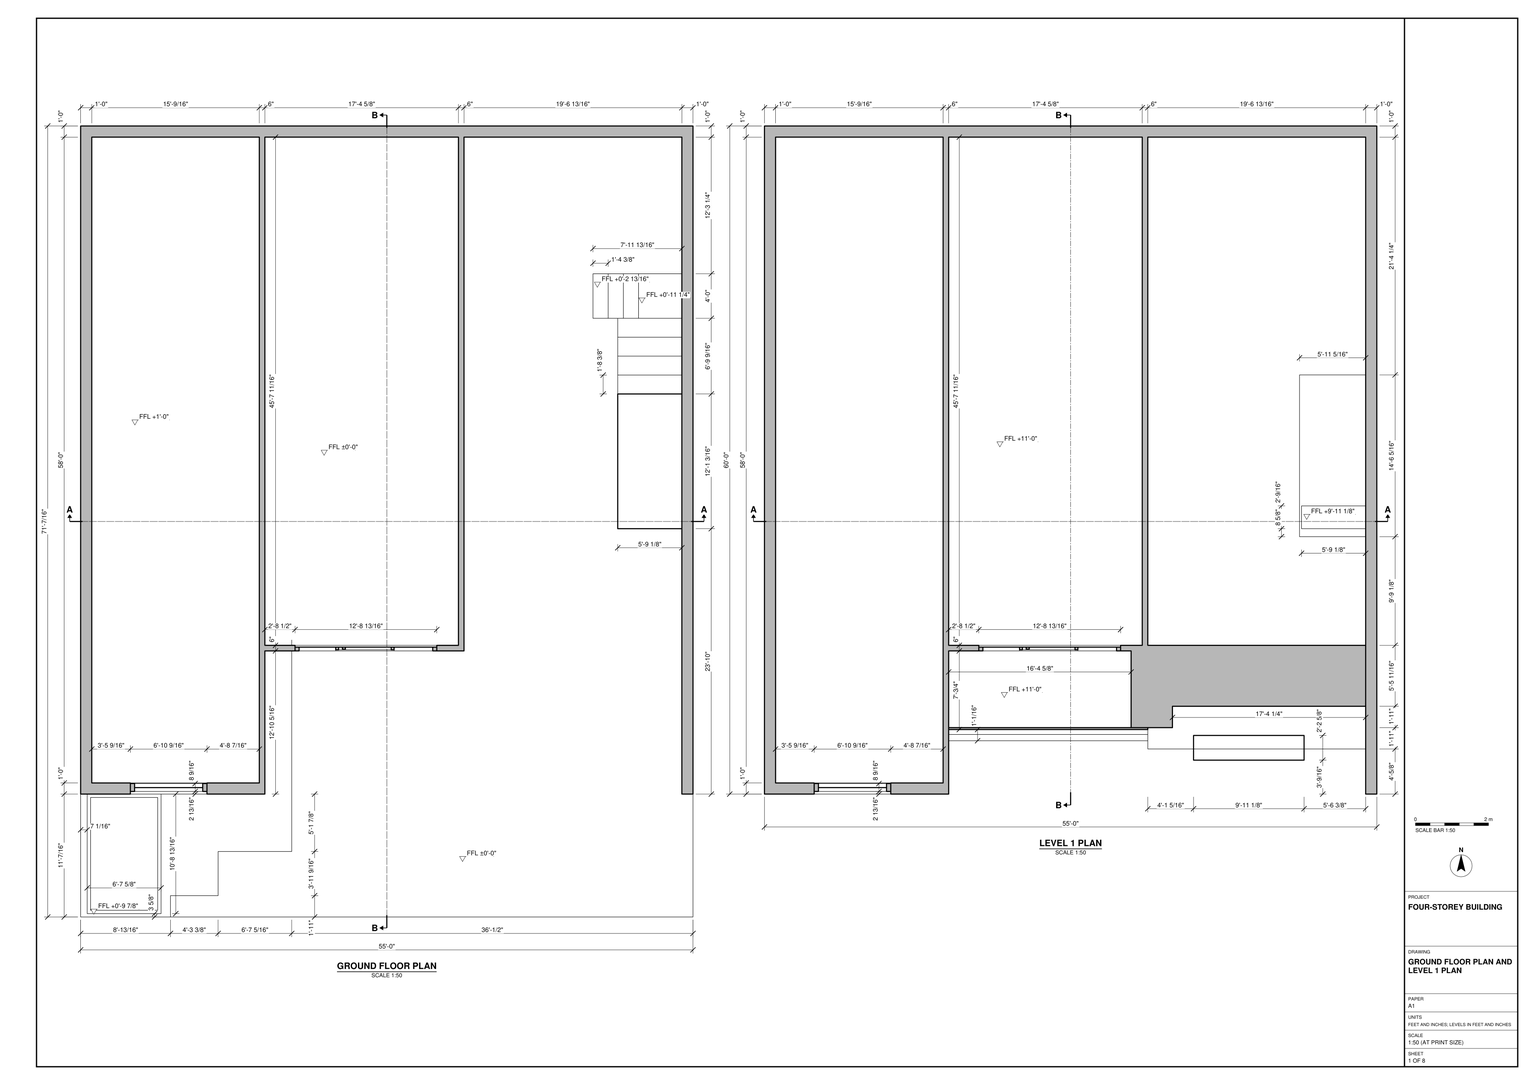
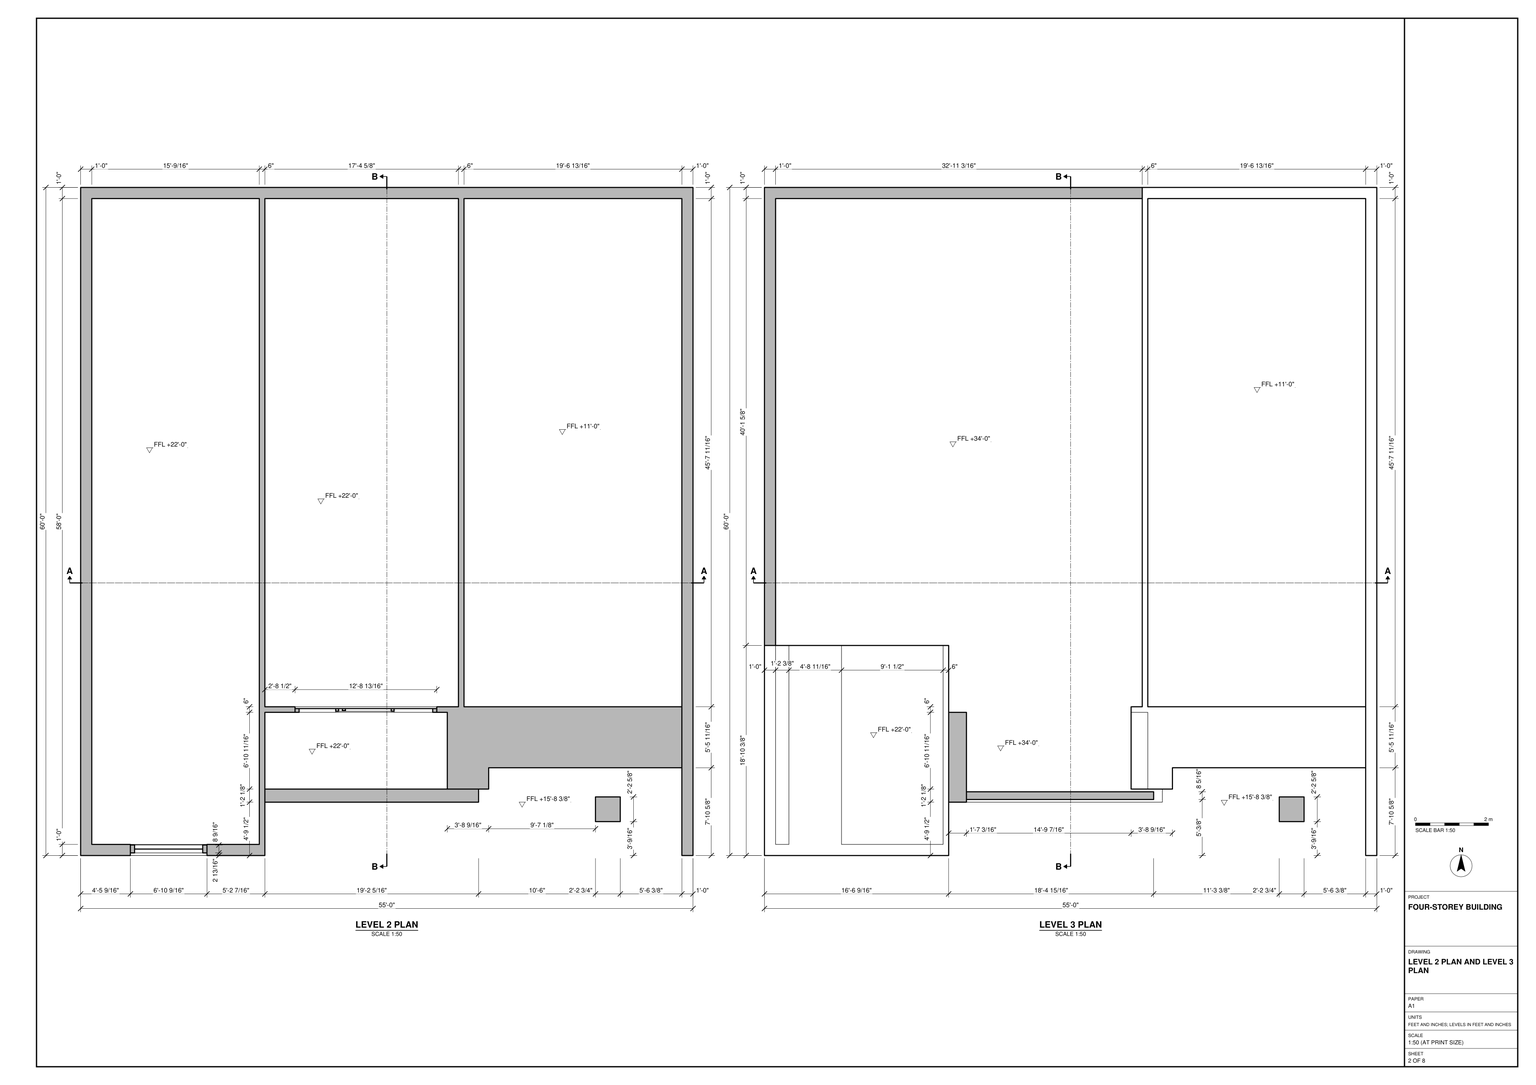
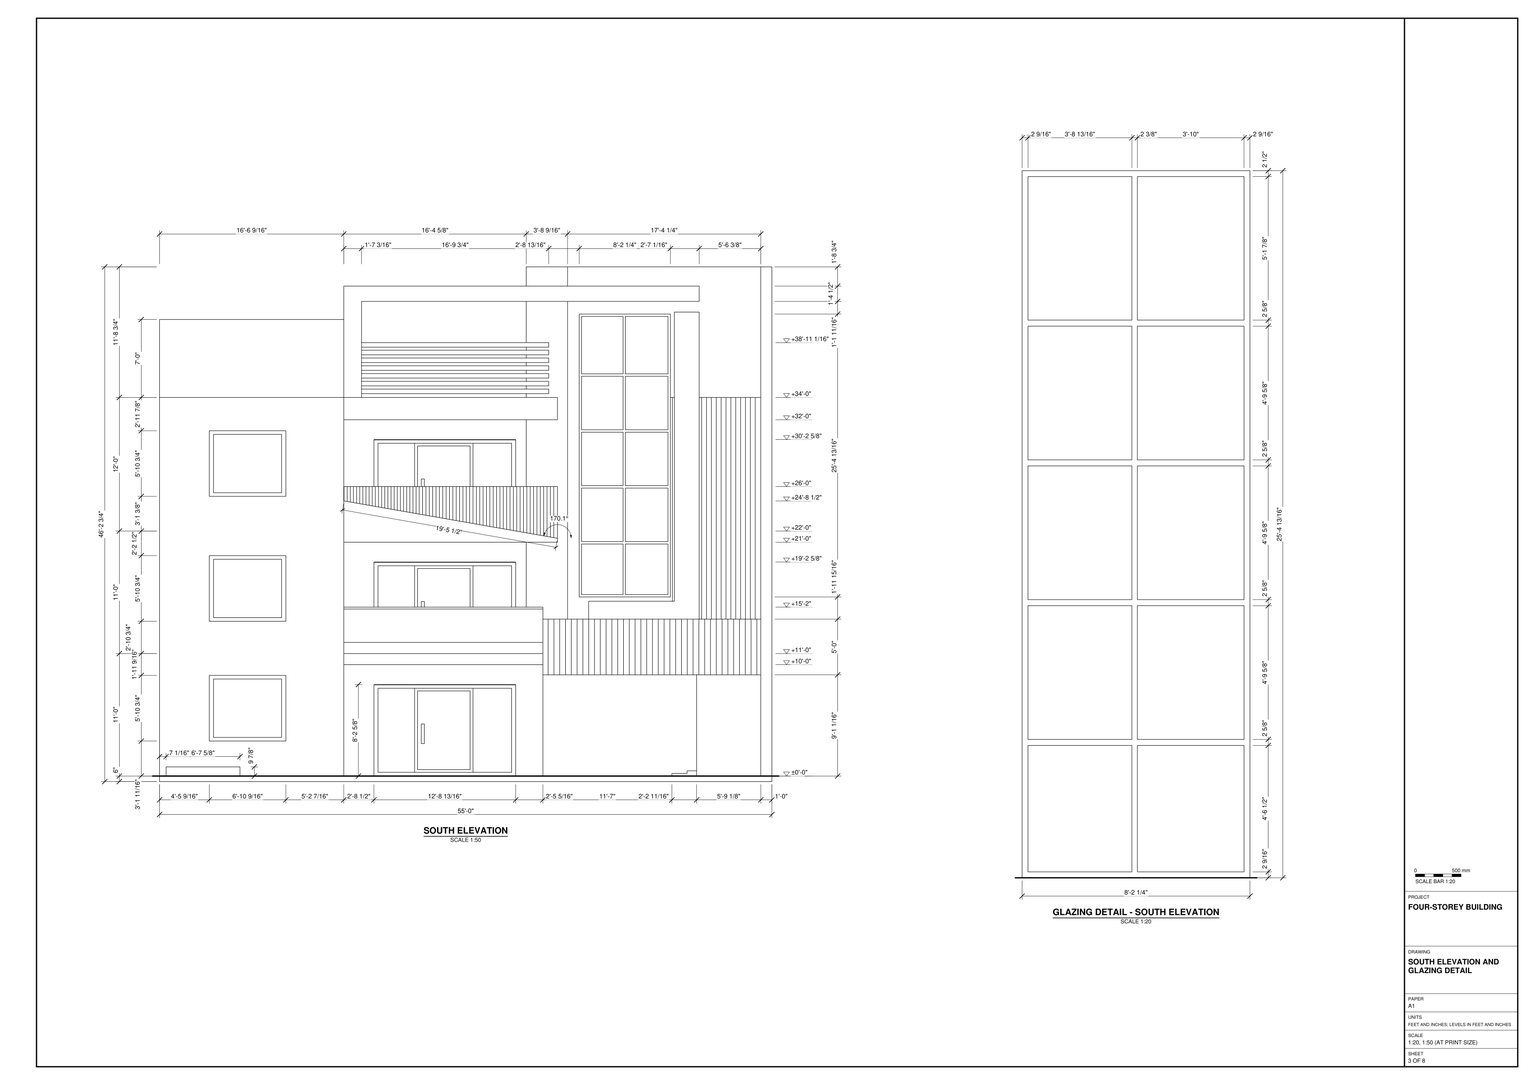
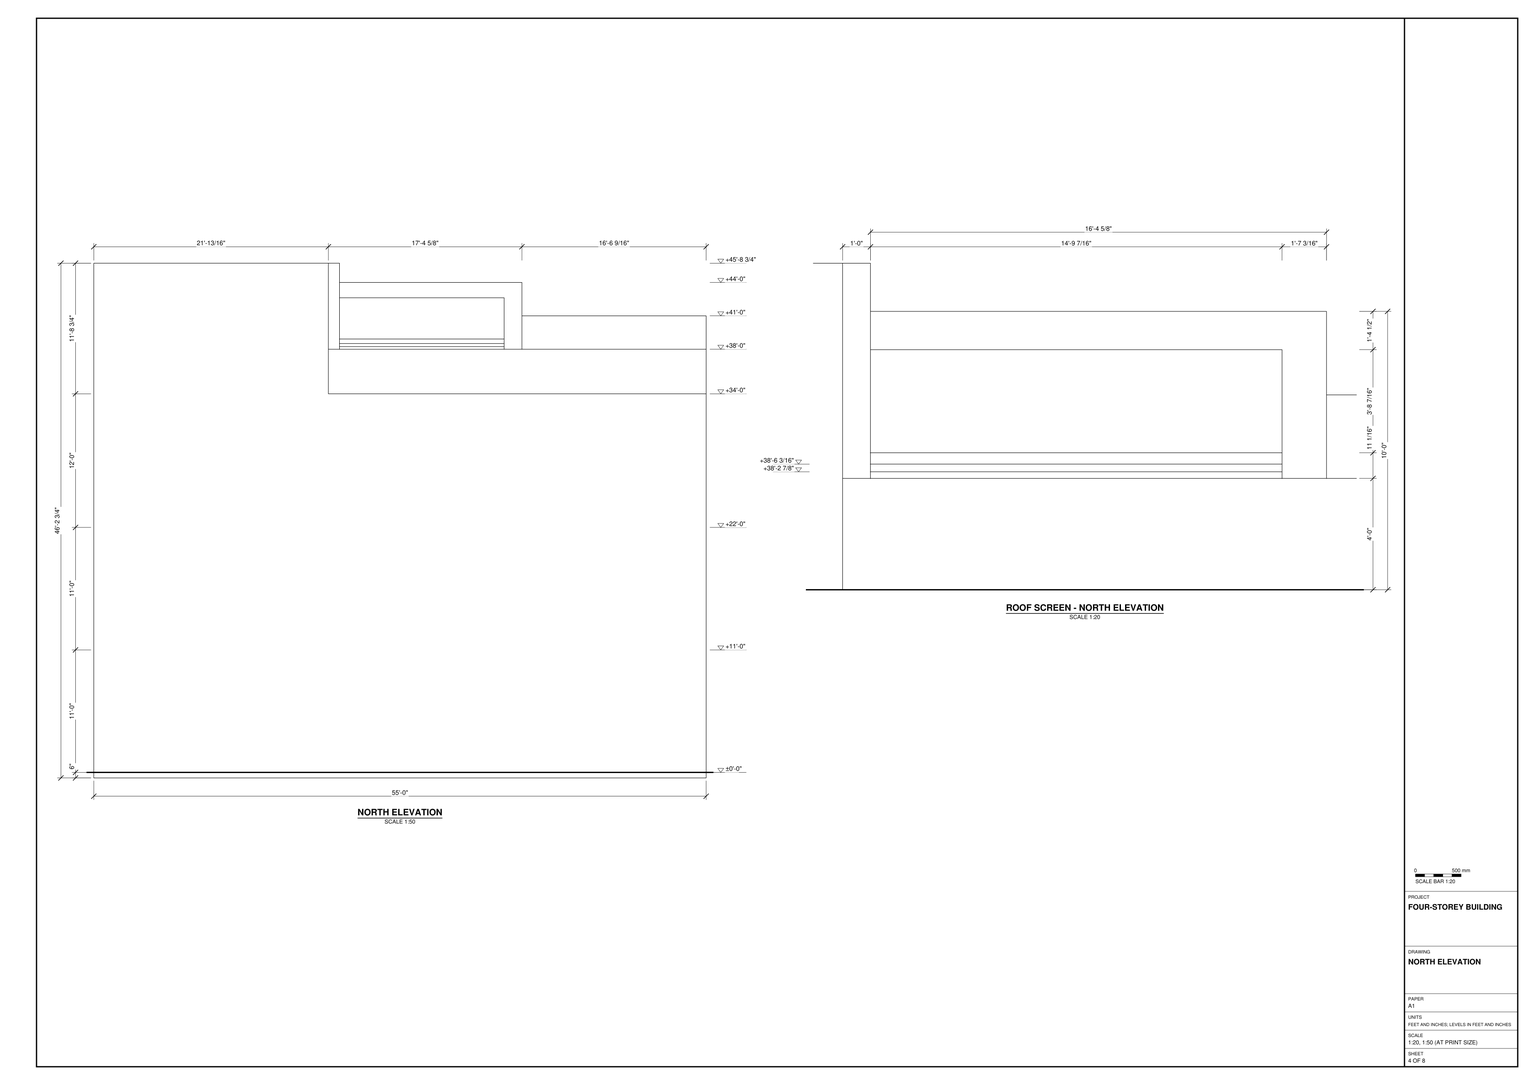
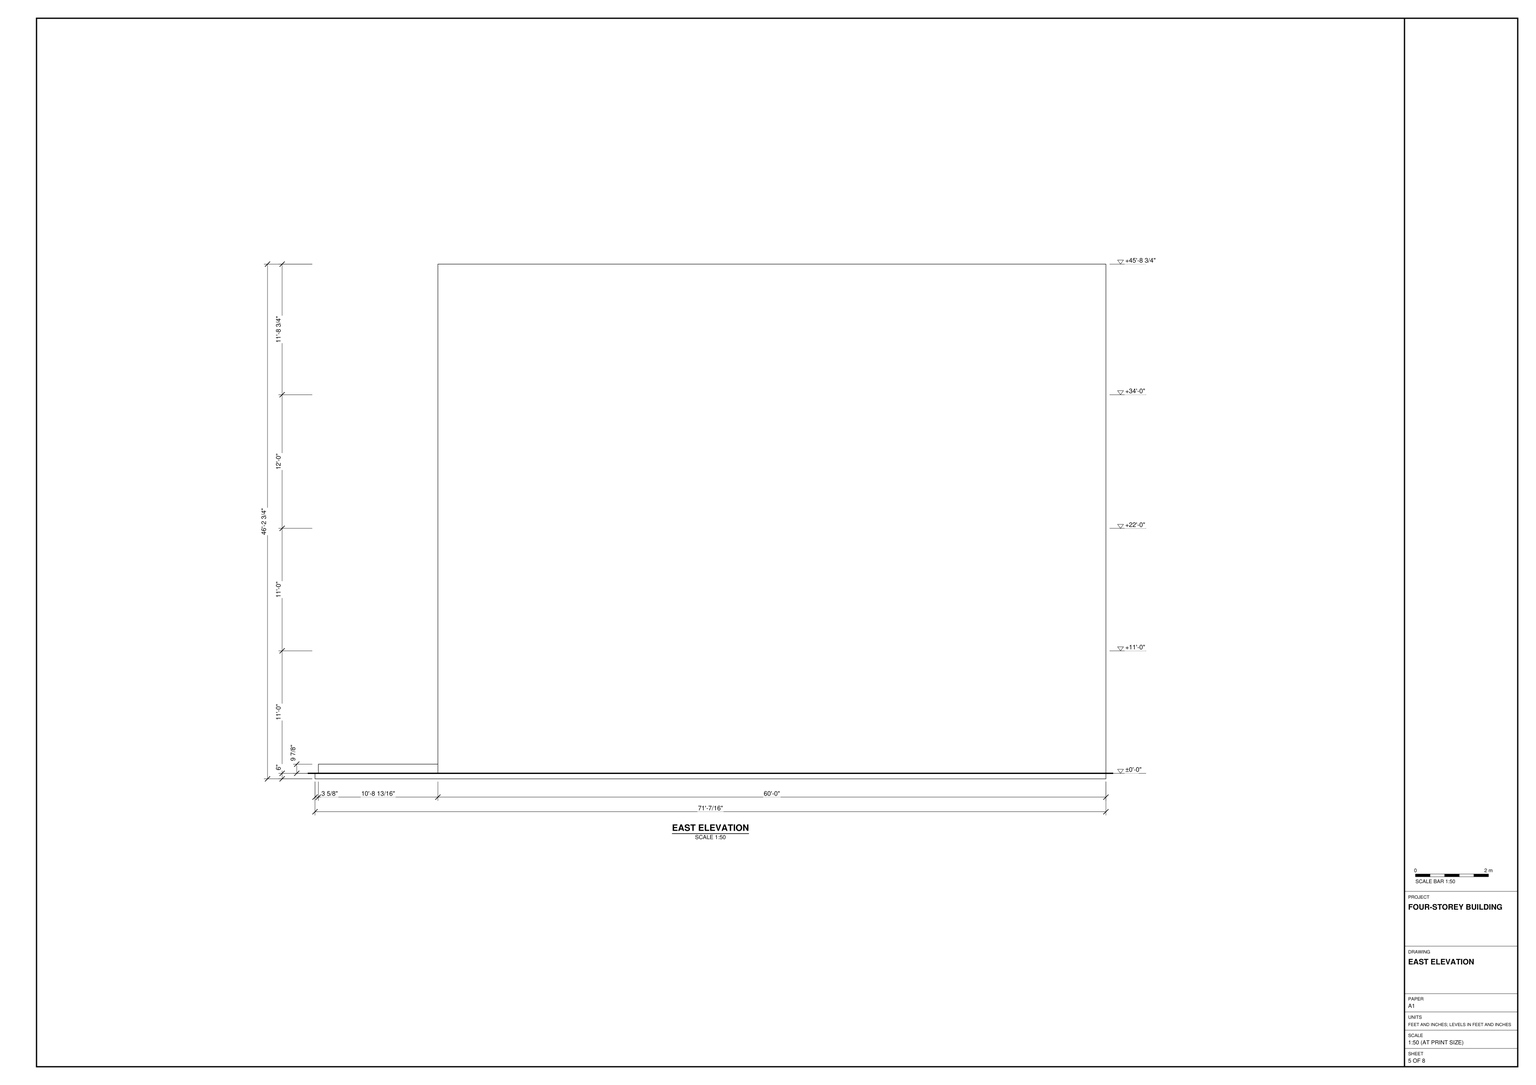
Build the four-storey building in SketchUp from task_files/diagram_01.pdf. Work in feet and inches. Including the approach on the south side, the model must measure 55'-0" wide by 71'-7/16" deep and 46'-2 3/4" high. Set the storey levels to ±0'-0", +11'-0", +22'-0" and +34'-0".

Use the floor plans to lay out the three longitudinal bays, with 1'-0" perimeter walls and 6" partitions where indicated. Follow each level's slab outline separately: the left bay projects beyond the central entrance, and the upper slabs stop short of the full footprint. Model the stepped approach, the stair and its landing in the right bay, and the flat roof sections at their respective heights.

Use the south elevation to place the stacked windows, glazed entrance and balcony doors. Include the balcony fronts and railings, the horizontal slats below the upper frame and the vertical screen on the right. Use the enlarged glazing detail for the frame and pane divisions of the tall window. Model built-in joinery and main furniture only where shown. Decor and loose items may be represented by any suitable library components.

Keep walls, slabs, roof sections and each furniture or joinery piece in separate groups or components, and use components for repeated parts. Save one SketchUp model as output_files/four_storey_building_balconies_and_multi_storey_glazing.skp.

# SketchUp Ruby script. Lengths in inches.
U = 1.inch
M = Sketchup.active_model
def pt(a) = Geom::Point3d.new(a.map { |v| v * U })
def face(e, loops, mat)
  f = e.add_face(loops[0].map { |a| pt(a) })
  loops[1..].each { |l| e.add_face(l.map { |a| pt(a) }).erase! }
  f.material = f.back_material = mat if mat
  f
end
# faces: each face lists its corners as indices into pts; further lists are holes
def faces(e, pts, list, mat = nil) = list.each { |f| face(e, (f[0].is_a?(Array) ? f : [f]).map { |l| l.map { |i| pts[i] } }, mat) }
# xy, xz, yz: faces in a plane at the given z, y or x. An outline is a flat list of corners, or four numbers for a rectangle; further outlines are holes
def ring(l) = l.size == 4 ? [[l[0], l[1]], [l[2], l[1]], [l[2], l[3]], [l[0], l[3]]] : l.each_slice(2).to_a
def flat(e, list, mat, &to3) = list.each { |f| face(e, (f[0].is_a?(Array) ? f : [f]).map { |l| ring(l).map { |u, v| to3.(u, v) } }, mat) }
def xy(e, z, list, mat = nil) = flat(e, list, mat) { |x, y| [x, y, z] }
def xz(e, y, list, mat = nil) = flat(e, list, mat) { |x, z| [x, y, z] }
def yz(e, x, list, mat = nil) = flat(e, list, mat) { |y, z| [x, y, z] }
def lines(e, pts, list) = list.each { |a, b| e.add_line(pt(pts[a]), pt(pts[b])) }
# prism: a flat outline (further loops are holes) pulled along v
def prism(e, loops, v, mat = nil)
  f = face(e, loops, mat); d = Geom::Vector3d.new(v.map { |x| x * U })
  f.pushpull(f.normal.samedirection?(d) ? d.length : -d.length)
end
def box(e, o, s, mat = nil) = prism(e, [[o, [o[0] + s[0], o[1], o[2]], [o[0] + s[0], o[1] + s[1], o[2]], [o[0], o[1] + s[1], o[2]]]], [0, 0, s[2]], mat)
def at(x, y, z, deg = 0) = Geom::Transformation.translation(pt([x, y, z])) * Geom::Transformation.rotation(ORIGIN, Z_AXIS, deg.degrees)
def axes(o, x, y, z) = Geom::Transformation.new([*x, 0, *y, 0, *z, 0, *pt(o).to_a, 1])
def part(name) = M.definitions.add(name)
# library, detail: a bought-in or finely detailed component or shape, given as its bounding box
def library(name, o, s) = part(name).tap { |d| box(d.entities, o, s) }
def detail(e, o, s) = box(e.add_group.entities, o, s)
def put(e, d, t, mat = nil) = e.add_instance(d, t).tap { |i| i.material = mat if mat }
def group(e, t, mat = nil) = e.add_group.tap { |g| g.transformation = t; g.material = mat if mat }.entities
root = M.entities
M.materials.add("[0043_SaddleBrown]").color = [97, 69, 19]
M.materials.add("[0043_SaddleBrown]1").color = [94, 69, 19]
M.materials.add("[0100_SteelBlue]").color = [76, 104, 180]
M.materials.add("[0100_SteelBlue]1").color = [113, 130, 180]
M.materials.add("[Asphalt Stamped Brick]").color = [149, 133, 134]
M.materials.add("[Blacktop Old 01]").color = [132, 136, 139]
M.materials.add("[Brick Tumbled]").color = [135, 132, 132]
M.materials.add("[Color C08]").color = [102, 51, 0]
M.materials.add("[Color M00]").color = [255, 255, 255]
M.materials.add("[Color M03]").color = [170, 170, 170]
M.materials.add("[Color M04]").color = [142, 142, 142]
M.materials.add("[Color M05]").color = [114, 114, 114]
M.materials.add("[Color M07]").color = [58, 58, 58]
M.materials.add("[Grass Light Green]").color = [138, 158, 69]
M.materials.add("[Metal Corrugated Shiny]").color = [193, 193, 193]
M.materials.add("[Metal Seamed]").color = [118, 119, 115]
M.materials.add("[Pavers with Grass Brick]").color = [187, 192, 176]
M.materials.add("[Translucent Glass Gray]").color = [128, 128, 128]
M.materials["[Translucent Glass Gray]"].alpha = 0.5
M.materials.add("[Wood Floor Dark]").color = [153, 94, 42]
c1 = part("Group\#3")
xy(c1.entities,0,[[0,0,90.625,11.375]],"[Color C08]")
xy(c1.entities,5.03,[[5.03,0,85.6,5.5],[5.03,5.5,85.6,11.375]],"[Color C08]")
xy(c1.entities,85.6,[[5.03,0,85.6,5.5],[5.03,5.5,85.6,11.375]],"[Color C08]")
xy(c1.entities,90.625,[[0,0,90.625,11.375]],"[Color C08]")
xz(c1.entities,0,[[[0,0,90.625,90.625],[5.03,5.03,85.6,85.6]]],"[Color C08]")
xz(c1.entities,5.5,[[5.03,5.03,85.6,85.6]],"[Translucent Glass Gray]")
xz(c1.entities,11.375,[[[0,0,90.625,90.625],[5.03,5.03,85.6,85.6]]],"[Color C08]")
yz(c1.entities,0,[[0,0,11.375,90.625]],"[Color C08]")
yz(c1.entities,5.03,[[0,5.03,5.5,85.6],[5.5,5.03,11.375,85.6]],"[Color C08]")
yz(c1.entities,85.6,[[0,5.03,5.5,85.6],[5.5,5.03,11.375,85.6]],"[Color C08]")
yz(c1.entities,90.625,[[0,0,11.375,90.625]],"[Color C08]")
c2 = part("Group\#4")
xy(c2.entities,0,[[0,0,236.9375,6.875]],"[Color C08]")
xy(c2.entities,6.8,[[6.8,0,67.98,6.875],[67.98,0,165.61,2.0625],[165.61,0,230.14,6.875],[67.98,2.0625,165.61,6.875]],"[Color C08]")
xy(c2.entities,11.7,[[72.88,2.0625,160.7,6.875]],"[Color C08]")
xy(c2.entities,59.36,[[79.14,3.0625,84.27,6.875]],"[Metal Corrugated Shiny]")
xy(c2.entities,95.11,[[79.14,3.0625,84.27,6.875]],"[Metal Corrugated Shiny]")
xy(c2.entities,155.42,[[72.88,2.0625,160.7,6.875]],"[Color C08]")
xy(c2.entities,160.33,[[6.8,0,67.98,6.875],[67.98,0,165.61,2.0625],[165.61,0,230.14,6.875],[67.98,2.0625,165.61,6.875]],"[Color C08]")
xy(c2.entities,167.125,[[0,0,236.9375,6.875]],"[Color C08]")
xz(c2.entities,0,[[[0,0,236.9375,167.125],[6.8,6.8,230.14,160.33]]],"[Color C08]")
xz(c2.entities,2.0625,[[[67.98,6.8,165.61,160.33],[72.88,11.7,160.7,155.42]]],"[Color C08]")
xz(c2.entities,3.0625,[[79.14,59.36,84.27,95.11]],"[Metal Corrugated Shiny]")
xz(c2.entities,6.875,[[[0,0,236.9375,167.125],[6.8,6.8,230.14,160.33]],[[67.98,6.8,165.61,160.33],[72.88,11.7,160.7,155.42]]],"[Color C08]")
xz(c2.entities,6.875,[[79.14,59.36,84.27,95.11]],"[Metal Corrugated Shiny]")
xz(c2.entities,6.875,[[6.8,6.8,67.98,160.33],[165.61,6.8,230.14,160.33],[[72.88,11.7,160.7,155.42],[79.14,59.36,84.27,95.11]]],"[Translucent Glass Gray]")
yz(c2.entities,0,[[0,0,6.875,167.125]],"[Color C08]")
yz(c2.entities,6.8,[[0,6.8,6.875,160.33]],"[Color C08]")
yz(c2.entities,67.98,[[2.0625,6.8,6.875,160.33]],"[Color C08]")
yz(c2.entities,72.88,[[2.0625,11.7,6.875,155.42]],"[Color C08]")
yz(c2.entities,79.14,[[3.0625,59.36,6.875,95.11]],"[Metal Corrugated Shiny]")
yz(c2.entities,84.27,[[3.0625,59.36,6.875,95.11]],"[Metal Corrugated Shiny]")
yz(c2.entities,160.7,[[2.0625,11.7,6.875,155.42]],"[Color C08]")
yz(c2.entities,165.61,[[2.0625,6.8,6.875,160.33]],"[Color C08]")
yz(c2.entities,230.14,[[0,6.8,6.875,160.33]],"[Color C08]")
yz(c2.entities,236.9375,[[0,0,6.875,167.125]],"[Color C08]")
xy(root,0,[[0,0,660,852.4375]])
xy(root,6,[[227.5,286.75,231.06,292.75],[198.5625,292.75,407.1875,840.4375]])
xy(root,6,[[96.8,0,660,0,660,132.4375,648,132.4375,648,840.4375,413.1875,840.4375,413.1875,286.75,383.85,286.75,383.85,292.75,231.06,292.75,231.06,286.75,227.5,286.75,227.5,70.5625,148.17,70.5625,148.17,23,96.8,23]],"[Blacktop Old 01]")
xy(root,6,[[[7.06,3.6,86.68,3.6,86.68,132.4375,198.5625,132.4375,198.5625,286.75,227.5,286.75,227.5,292.75,198.5625,292.75,198.5625,840.4375,407.1875,840.4375,407.1875,292.75,383.85,292.75,383.85,286.75,413.1875,286.75,413.1875,840.4375,648,840.4375,648,132.4375,660,132.4375,660,852.4375,0,852.4375,0,132.4375,7.06,132.4375],[10.7,7.25,83.04,128.79]],[10.7,7.25,83.04,128.79]],"[Grass Light Green]")
xy(root,6,[[0,0,96.8,0,96.8,23,148.17,23,148.17,70.5625,227.5,70.5625,227.5,286.75,198.5625,286.75,198.5625,132.4375,86.68,132.4375,86.68,3.6,7.06,3.6,7.06,132.4375,0,132.4375]],"[Pavers with Grass Brick]")
xy(root,15.875,[[[7.06,3.6,86.68,132.4375],[10.7,7.25,83.04,128.79]]],"[Asphalt Stamped Brick]")
xy(root,18,[[12,144.4375,192.5625,840.4375]])
xy(root,43.71,[[53.59,132.4375,136.15,144.4375]])
xy(root,104.24,[[231.06,286.75,383.85,292.75]])
xy(root,114.46,[[53.59,132.4375,136.15,144.4375]])
xy(root,115.0625,[[413.1875,181.0625,413.1875,840.4375,648,840.4375,648,584.17,576.7,584.17,576.7,409.86,648,409.86,648,181.0625]])
xy(root,126,[[198.5625,189.9375,413.1875,286.75]])
xy(root,127.1875,[[198.5625,292.75,407.1875,840.4375]])
xy(root,132,[[12,144.4375,192.5625,840.4375]])
xy(root,138,[[12,144.4375,192.5625,840.4375],[198.5625,196.6875,413.1875,204.0625],[198.5625,204.0625,395.18,286.75],[231.06,286.75,383.85,292.75],[198.5625,292.75,407.1875,840.4375],
  [413.1875,292.75,648,292.75,648,409.86,576.7,409.86,576.7,584.17,648,584.17,648,840.4375,413.1875,840.4375]])
xy(root,138,[[198.5625,189.9375,413.1875,196.6875]],"[Color M00]")
xy(root,150,[[198.5625,202,413.1875,204.0625]])
xy(root,150,[[198.5625,196.6875,413.1875,202]],"[Color M05]")
xy(root,172.77,[[53.59,132.4375,136.15,144.4375]])
xy(root,175.0625,[[462.48,169,581.61,181.0625],[462.48,181.0625,581.61,195.625]])
xy(root,175.0625,[[413.1875,181.0625,462.48,181.0625,462.48,195.625,581.61,195.625,581.61,181.0625,648,181.0625,648,227.0625,439.75,227.0625,439.75,204.0625,413.1875,204.0625]],"[Wood Floor Dark]")
xy(root,186,[[198.5625,202,413.1875,204.0625]])
xy(root,188,[[198.5625,202,413.1875,204.0625]],"[Metal Seamed]")
xy(root,194.375,[[462.48,169,554.87,195.625]])
xy(root,236.24,[[231.06,286.75,383.85,292.75]])
xy(root,243.52,[[53.59,132.4375,136.15,144.4375]])
xy(root,258,[[198.5625,189.9375,198.5625,286.75,216.82,286.75,216.82,213.125,378.07,213.125,378.07,286.75,395.18,286.75,395.18,204.0625,428.875,204.0625,428.875,189.9375],[395.18,204.0625,413.1875,286.75]])
xy(root,258,[[216.82,213.125,378.07,286.75]],"[Color M07]")
xy(root,264,[[12,144.4375,192.5625,840.4375],[198.5625,292.75,407.1875,840.4375]])
xy(root,270,[[12,144.4375,192.5625,840.4375],[198.5625,204.0625,395.18,286.75],[395.18,204.0625,413.1875,286.75],[231.06,286.75,383.85,292.75],[198.5625,292.75,407.1875,840.4375]])
xy(root,307.4,[[53.59,132.4375,136.15,144.4375]])
xy(root,318,[[198.5625,189.9375,428.875,204.0625]])
xy(root,368.24,[[231.06,286.75,383.85,292.75]])
xy(root,378.15,[[53.59,132.4375,136.15,144.4375]])
xy(root,390,[[198.5625,189.9375,198.5625,286.75,395.18,286.75,395.18,204.0625,428.875,204.0625,428.875,189.9375],[395.18,204.0625,413.1875,286.75]])
xy(root,400.875,[[12,144.4375,192.5625,840.4375]])
xy(root,408,[[198.5625,292.75,407.1875,840.4375]])
xy(root,414,[[0,132.4375,0,358.8125,12,358.8125,12,144.4375,26.375,144.4375,26.375,358.8125,83.0625,358.8125,83.0625,144.4375,192.5625,144.4375,192.5625,358.8125,198.5625,358.8125,198.5625,132.4375],[217.73,189.9375,428.875,189.9375,428.875,204.0625,395.18,204.0625,395.18,292.75,407.1875,292.75,407.1875,840.4375,12,840.4375,12,358.8125,198.5625,358.8125,198.5625,286.75,217.73,286.75],[198.5625,189.9375,217.73,286.75],[395.18,204.0625,413.1875,286.75],[0,358.8125,12,852.4375],
  [12,840.4375,407.1875,852.4375]])
xy(root,418.11,[[217.73,192.82,419.48,201.14]],"[0043_SaddleBrown]1")
xy(root,422.99,[[217.73,192.82,419.48,201.14]],"[0043_SaddleBrown]1")
xy(root,426.49,[[217.73,192.82,419.48,201.14]],"[0043_SaddleBrown]1")
xy(root,431.36,[[217.73,192.82,419.48,201.14]],"[0043_SaddleBrown]1")
xy(root,434.86,[[217.73,192.82,419.48,201.14]],"[0043_SaddleBrown]1")
xy(root,439.74,[[217.73,192.82,419.48,201.14]],"[0043_SaddleBrown]1")
xy(root,443.24,[[217.73,192.82,419.48,201.14]],"[0043_SaddleBrown]1")
xy(root,448.11,[[217.73,192.82,419.48,201.14]],"[0043_SaddleBrown]1")
xy(root,451.61,[[217.73,192.82,419.48,201.14]],"[0043_SaddleBrown]1")
xy(root,456.49,[[217.73,192.82,419.48,201.14]],"[0043_SaddleBrown]1")
xy(root,459.99,[[217.73,192.82,419.48,201.14]],"[0043_SaddleBrown]1")
xy(root,462,[[0,358.8125,12,358.8125,12,840.4375,407.1875,840.4375,407.1875,852.4375,0,852.4375]],"[Color M03]")
xy(root,464.86,[[217.73,192.82,419.48,201.14]],"[0043_SaddleBrown]1")
xy(root,468.17,[[217.73,192.82,419.48,201.14]],"[0043_SaddleBrown]1")
xy(root,473.05,[[217.73,192.82,419.48,201.14]],"[0043_SaddleBrown]1")
xy(root,498,[[0,132.4375,198.5625,358.8125]],"[0100_SteelBlue]1")
xy(root,506,[[554.87,169,581.61,195.625]])
xy(root,517.49,[[[217.73,189.9375,217.73,286.75,395.18,286.75,395.18,204.0625,439.75,204.0625,439.75,227.0625,581.61,227.0625,581.61,189.9375],[227.26,213.58,236.33,270.02],[245.01,213.58,254.08,270.02],[262.76,213.58,271.83,270.02],[280.51,213.58,289.58,270.02],[298.26,213.58,307.33,270.02],[316.01,213.58,325.08,270.02],[333.26,213.58,342.33,270.02],[349.83,213.58,358.89,270.02]],[395.18,204.0625,407.1875,286.75],[407.1875,204.0625,439.75,227.0625]])
xy(root,534,[[[198.5625,189.9375,581.61,189.9375,581.61,227.0625,439.75,227.0625,439.75,204.0625,395.18,204.0625,395.18,286.75,198.5625,286.75],[227.26,213.58,236.33,270.02],[245.01,213.58,254.08,270.02],[262.76,213.58,271.83,270.02],[280.51,213.58,289.58,270.02],[298.26,213.58,307.33,270.02],[316.01,213.58,325.08,270.02],[333.26,213.58,342.33,270.02],[349.83,213.58,358.89,270.02]],[395.18,204.0625,407.1875,286.75],[407.1875,204.0625,439.75,227.0625]])
xy(root,548.75,[[413.1875,292.75,648,840.4375]])
xy(root,554.75,[[648,132.4375,660,132.4375,660,852.4375,407.1875,852.4375,407.1875,292.75,395.18,292.75,395.18,204.0625,439.75,204.0625,439.75,227.0625,648,227.0625]],"[Color M04]")
xz(root,0,[[0,0,660,6]])
xz(root,3.6,[[7.06,6,86.68,15.875]],"[Asphalt Stamped Brick]")
xz(root,7.25,[[10.7,6,83.04,15.875]],"[Asphalt Stamped Brick]")
xz(root,128.79,[[10.7,6,83.04,15.875]],"[Asphalt Stamped Brick]")
xz(root,132.4375,[[648,6,660,554.75]])
xz(root,132.4375,[[0,414,198.5625,498]],"[0100_SteelBlue]1")
xz(root,132.4375,[[[0,6,7.06,6,7.06,15.875,86.68,15.875,86.68,6,198.5625,6,198.5625,414,0,414],[53.59,43.71,136.15,114.46],[53.59,307.4,136.15,378.15],[53.59,172.77,136.15,243.52]]],"[Brick Tumbled]")
xz(root,144.4375,[[[12,18,192.5625,126],[53.59,43.71,136.15,114.46]],[12,126,192.5625,132],[12,132,192.5625,138],[[12,138,192.5625,258],[53.59,172.77,136.15,243.52]],[12,258,192.5625,264],
  [12,264,192.5625,270],[[12,270,192.5625,390],[53.59,307.4,136.15,378.15]],[12,390,192.5625,400.875]])
xz(root,169,[[462.48,175.0625,581.61,175.0625,581.61,506,554.87,506,554.87,194.375,462.48,194.375]])
xz(root,181.0625,[[648,126,650.04,138],[650.04,126,656.29,138]])
xz(root,181.0625,[[413.1875,115.0625,418.79,175.0625],[418.79,115.0625,425.04,175.0625],[425.04,115.0625,431.29,175.0625],[431.29,115.0625,437.54,175.0625],[437.54,115.0625,443.79,175.0625],
  [443.79,115.0625,450.04,175.0625],[450.04,115.0625,456.29,175.0625],[456.29,115.0625,462.54,175.0625],[462.54,115.0625,468.79,175.0625],[468.79,115.0625,475.04,175.0625],
  [475.04,115.0625,481.29,175.0625],[481.29,115.0625,487.54,175.0625],[487.54,115.0625,493.79,175.0625],[493.79,115.0625,500.04,175.0625],[500.04,115.0625,506.29,175.0625],
  [506.29,115.0625,512.54,175.0625],[512.54,115.0625,518.79,175.0625],[518.79,115.0625,525.04,175.0625],[525.04,115.0625,531.29,175.0625],[531.29,115.0625,537.54,175.0625],
  [537.54,115.0625,543.79,175.0625],[543.79,115.0625,550.04,175.0625],[550.04,115.0625,556.29,175.0625],[556.29,115.0625,562.54,175.0625],[562.54,115.0625,568.79,175.0625],
  [568.79,115.0625,575.04,175.0625],[575.04,115.0625,581.29,175.0625],[581.29,115.0625,587.54,175.0625],[587.54,115.0625,593.79,175.0625],[593.79,115.0625,600.04,175.0625],
  [600.04,115.0625,606.29,175.0625],[606.29,115.0625,612.54,175.0625],[612.54,115.0625,618.79,175.0625],[618.79,115.0625,625.04,175.0625],[625.04,115.0625,631.29,175.0625],
  [631.29,115.0625,637.54,175.0625],[637.54,115.0625,643.79,175.0625],[643.79,115.0625,648,175.0625]],"[Wood Floor Dark]")
xz(root,189.9375,[[198.5625,126,413.1875,138],[198.5625,258,428.875,258,428.875,262.23,428.08,262.37,424.87,262.93,421.24,263.56,417.62,264.2,413.99,264.83,410.37,265.47,406.74,266.1,403.12,266.74,399.49,267.37,395.87,268,392.24,268.64,388.62,269.27,384.99,269.91,381.37,270.54,377.74,271.17,374.12,271.81,370.49,272.44,366.87,273.08,363.24,273.71,359.62,274.35,355.99,274.98,352.37,275.61,348.74,276.25,345.12,276.88,341.49,277.52,337.87,278.15,334.24,278.79,330.62,279.42,326.99,280.05,323.37,280.6875,319.74,281.32,316.12,281.96,312.49,282.59,308.87,283.22,305.24,283.86,301.62,284.49,297.99,285.13,294.37,285.76,290.74,286.4,287.12,287.03,283.49,287.66,279.87,288.3,276.49,288.89,273.12,289.48,269.74,290.07,266.37,290.66,262.99,291.25,259.62,291.84,256.24,292.43,252.87,293.02,249.49,293.61,246.12,294.2,242.74,294.79,239.37,295.38,235.99,295.97,232.62,296.56,229.24,297.16,225.87,297.75,222.49,298.34,219.12,298.93,215.74,299.52,212.37,300.11,208.99,300.7,205.62,301.29,202.24,301.88,198.87,302.47,198.5625,302.52],[198.5625,390,428.875,414],[198.5625,414,217.73,414,217.73,517.49,581.61,517.49,581.61,534,198.5625,534]])
xz(root,189.9375,[[428.875,262.23,428.875,318,424.87,318,424.87,262.93,428.08,262.37],[424.87,262.93,424.87,318,421.24,318,421.24,263.56],[421.24,263.56,421.24,318,417.62,318,417.62,264.2],[417.62,264.2,417.62,318,413.99,318,413.99,264.83],[413.99,264.83,413.99,318,410.37,318,410.37,265.47],
  [410.37,265.47,410.37,318,406.74,318,406.74,266.1],[406.74,266.1,406.74,318,403.12,318,403.12,266.74],[403.12,266.74,403.12,318,399.49,318,399.49,267.37],[399.49,267.37,399.49,318,395.87,318,395.87,268],[395.87,268,395.87,318,392.24,318,392.24,268.64],
  [392.24,268.64,392.24,318,388.62,318,388.62,269.27],[388.62,269.27,388.62,318,384.99,318,384.99,269.91],[384.99,269.91,384.99,318,381.37,318,381.37,270.54],[381.37,270.54,381.37,318,377.74,318,377.74,271.17],[377.74,271.17,377.74,318,374.12,318,374.12,271.81],
  [374.12,271.81,374.12,318,370.49,318,370.49,272.44],[370.49,272.44,370.49,318,366.87,318,366.87,273.08],[366.87,273.08,366.87,318,363.24,318,363.24,273.71],[363.24,273.71,363.24,318,359.62,318,359.62,274.35],[359.62,274.35,359.62,318,355.99,318,355.99,274.98],
  [355.99,274.98,355.99,318,352.37,318,352.37,275.61],[352.37,275.61,352.37,318,348.74,318,348.74,276.25],[348.74,276.25,348.74,318,345.12,318,345.12,276.88],[345.12,276.88,345.12,318,341.49,318,341.49,277.52],[341.49,277.52,341.49,318,337.87,318,337.87,278.15],
  [337.87,278.15,337.87,318,334.24,318,334.24,278.79],[334.24,278.79,334.24,318,330.62,318,330.62,279.42],[330.62,279.42,330.62,318,326.99,318,326.99,280.05],[326.99,280.05,326.99,318,323.37,318,323.37,280.6875],[323.37,280.6875,323.37,318,319.74,318,319.74,281.32],
  [319.74,281.32,319.74,318,316.12,318,316.12,281.96],[316.12,281.96,316.12,318,312.49,318,312.49,282.59],[312.49,282.59,312.49,318,308.87,318,308.87,283.22],[308.87,283.22,308.87,318,305.24,318,305.24,283.86],[305.24,283.86,305.24,318,301.62,318,301.62,284.49],
  [301.62,284.49,301.62,318,297.99,318,297.99,285.13],[297.99,285.13,297.99,318,294.37,318,294.37,285.76],[294.37,285.76,294.37,318,290.74,318,290.74,286.4],[290.74,286.4,290.74,318,287.12,318,287.12,287.03],[287.12,287.03,287.12,318,283.49,318,283.49,287.66],
  [283.49,287.66,283.49,318,279.87,318,279.87,288.3],[279.87,288.3,279.87,318,276.49,318,276.49,288.89],[276.49,288.89,276.49,318,273.12,318,273.12,289.48],[273.12,289.48,273.12,318,269.74,318,269.74,290.07],[269.74,290.07,269.74,318,266.37,318,266.37,290.66],
  [266.37,290.66,266.37,318,262.99,318,262.99,291.25],[262.99,291.25,262.99,318,259.62,318,259.62,291.84],[259.62,291.84,259.62,318,256.24,318,256.24,292.43],[256.24,292.43,256.24,318,252.87,318,252.87,293.02],[252.87,293.02,252.87,318,249.49,318,249.49,293.61],
  [249.49,293.61,249.49,318,246.12,318,246.12,294.2],[246.12,294.2,246.12,318,242.74,318,242.74,294.79],[242.74,294.79,242.74,318,239.37,318,239.37,295.38],[239.37,295.38,239.37,318,235.99,318,235.99,295.97],[235.99,295.97,235.99,318,232.62,318,232.62,296.56],
  [232.62,296.56,232.62,318,229.24,318,229.24,297.16],[229.24,297.16,229.24,318,225.87,318,225.87,297.75],[225.87,297.75,225.87,318,222.49,318,222.49,298.34],[222.49,298.34,222.49,318,219.12,318,219.12,298.93],[219.12,298.93,219.12,318,215.74,318,215.74,299.52],
  [215.74,299.52,215.74,318,212.37,318,212.37,300.11],[212.37,300.11,212.37,318,208.99,318,208.99,300.7],[208.99,300.7,208.99,318,205.62,318,205.62,301.29],[205.62,301.29,205.62,318,202.24,318,202.24,301.88],[202.24,301.88,202.24,318,198.87,318,198.87,302.47],
  [198.87,302.47,198.87,318,198.5625,318,198.5625,302.52]],"[Wood Floor Dark]")
xz(root,192.82,[[217.73,418.11,419.48,422.99],[217.73,426.49,419.48,431.36],[217.73,434.86,419.48,439.74],[217.73,443.24,419.48,448.11],[217.73,451.61,419.48,456.49],
  [217.73,459.99,419.48,464.86],[217.73,468.17,419.48,473.05]],"[0043_SaddleBrown]1")
xz(root,195.625,[[462.48,175.0625,462.48,194.375,554.87,194.375,554.87,506,581.61,506,581.61,175.0625]])
xz(root,196.6875,[[198.5625,138,413.1875,150]],"[Color M05]")
xz(root,201.14,[[217.73,418.11,419.48,422.99],[217.73,426.49,419.48,431.36],[217.73,434.86,419.48,439.74],[217.73,443.24,419.48,448.11],[217.73,451.61,419.48,456.49],
  [217.73,459.99,419.48,464.86],[217.73,468.17,419.48,473.05]],"[0043_SaddleBrown]1")
xz(root,202,[[198.5625,186,413.1875,188]],"[Metal Seamed]")
xz(root,202,[[198.5625,150,413.1875,186]],"[Translucent Glass Gray]")
xz(root,204.0625,[[198.5625,138,395.18,150],[395.18,138,413.1875,150],[395.18,150,413.1875,186],[395.18,186,413.1875,188],[413.1875,258,428.875,270],
  [198.5625,270,395.18,318],[395.18,270,413.1875,318],[413.1875,270,428.875,318],[413.1875,390,428.875,414]])
xz(root,204.0625,[[413.1875,175.0625,439.75,175.0625,439.75,517.49,395.18,517.49,395.18,414,428.875,414,428.875,390,395.18,390,395.18,318,428.875,318,428.875,258,395.18,258,395.18,188,413.1875,188],[395.18,534,439.75,554.75]],"[0100_SteelBlue]")
xz(root,204.0625,[[198.5625,186,395.18,188]],"[Metal Seamed]")
xz(root,204.0625,[[198.5625,150,395.18,186]],"[Translucent Glass Gray]")
xz(root,213.58,[[227.26,517.49,236.33,534],[245.01,517.49,254.08,534],[262.76,517.49,271.83,534],[280.51,517.49,289.58,534],[298.26,517.49,307.33,534],
  [316.01,517.49,325.08,534],[333.26,517.49,342.33,534],[349.83,517.49,358.89,534]])
xz(root,227.0625,[[454.85,135.57,548,138.17],[407.1875,517.49,413.1875,534],[413.1875,517.49,581.61,534]])
xz(root,227.0625,[[439.75,175.0625,552.77,175.0625,552.77,414,550.55,414,550.55,199.02,452.3,199.02,452.3,503.83,550.55,503.83,550.55,414,648,414,648,554.75,439.75,554.75,439.75,534,581.61,534,581.61,517.49,439.75,517.49]],"[0100_SteelBlue]")
xz(root,227.0625,[[[452.3,199.02,550.55,503.83],[502.02,439.42,548,501.28],[454.85,439.42,499.65,501.28],[502.02,258.67,548,316.32],[502.02,318.92,548,376.57],[502.02,379.17,548,436.82],[454.85,258.67,499.65,316.32],[454.85,318.92,499.65,376.57],[454.85,379.17,499.65,436.82],[502.02,201.57,548,256.07],[454.85,201.57,499.65,256.07]]],"[Color M07]")
xz(root,227.0625,[[454.85,201.57,499.65,256.07],[502.02,201.57,548,256.07],[454.85,258.67,499.65,316.32],[502.02,258.67,548,316.32],[454.85,318.92,499.65,376.57],
  [502.02,318.92,548,376.57],[454.85,379.17,499.65,436.82],[502.02,379.17,548,436.82],[454.85,439.42,499.65,501.28],[502.02,439.42,548,501.28]],"[Translucent Glass Gray]")
xz(root,227.0625,[[552.77,175.0625,558.02,414],[558.02,175.0625,563.27,414],[563.27,175.0625,568.52,414],[568.52,175.0625,573.77,414],[573.77,175.0625,579.02,414],
  [579.02,175.0625,584.27,414],[584.27,175.0625,589.52,414],[589.52,175.0625,594.77,414],[594.77,175.0625,600.02,414],[600.02,175.0625,605.27,414],
  [605.27,175.0625,610.52,414],[610.52,175.0625,615.77,414],[615.77,175.0625,621.02,414],[621.02,175.0625,626.27,414],[626.27,175.0625,631.52,414],
  [631.52,175.0625,636.77,414],[636.77,175.0625,642.02,414],[642.02,175.0625,648,414]],"[Wood Floor Dark]")
xz(root,270.02,[[227.26,517.49,236.33,534],[245.01,517.49,254.08,534],[262.76,517.49,271.83,534],[280.51,517.49,289.58,534],[298.26,517.49,307.33,534],
  [316.01,517.49,325.08,534],[333.26,517.49,342.33,534],[349.83,517.49,358.89,534]])
xz(root,286.75,[[198.5625,6,231.06,6,231.06,104.24,383.85,104.24,383.85,6,413.1875,6,413.1875,126,198.5625,126],[198.5625,126,395.18,138],[395.18,126,413.1875,138],[198.5625,138,231.06,138,231.06,236.24,383.85,236.24,383.85,138,395.18,138,395.18,258,198.5625,258],[198.5625,258,395.18,270],
  [395.18,258,413.1875,270],[198.5625,270,231.06,270,231.06,368.24,383.85,368.24,383.85,270,395.18,270,395.18,390,198.5625,390],[198.5625,414,198.5625,534,395.18,534,395.18,517.49,217.73,517.49,217.73,414],[395.18,517.49,407.1875,534]])
xz(root,292.75,[[198.5625,6,198.5625,126,407.1875,126,407.1875,6,383.85,6,383.85,104.24,231.06,104.24,231.06,6],[198.5625,126,407.1875,127.1875],[198.5625,127.1875,231.06,138],[231.06,127.1875,383.85,138],[383.85,127.1875,407.1875,138],
  [198.5625,138,198.5625,258,407.1875,258,407.1875,138,383.85,138,383.85,236.24,231.06,236.24,231.06,138],[413.1875,138,648,548.75],[198.5625,258,407.1875,264],[198.5625,264,231.06,270],[231.06,264,383.85,270],
  [383.85,264,407.1875,270],[198.5625,270,198.5625,390,407.1875,390,407.1875,270,383.85,270,383.85,368.24,231.06,368.24,231.06,270],[198.5625,390,407.1875,408],[395.18,408,407.1875,414],[395.18,414,407.1875,554.75]])
xz(root,358.8125,[[0,414,12,462]])
xz(root,358.8125,[[12,414,12,462,0,462,0,498,198.5625,498,198.5625,414]],"[0100_SteelBlue]1")
xz(root,409.86,[[576.7,115.0625,648,138]])
xz(root,584.17,[[576.7,115.0625,648,138]])
xz(root,840.4375,[[198.5625,6,407.1875,126],[413.1875,6,648,115.0625],[12,18,192.5625,126],[413.1875,115.0625,648,126],[12,126,192.5625,132],
  [198.5625,126,407.1875,127.1875],[413.1875,126,648,138],[198.5625,127.1875,250.9,138],[250.9,127.1875,261.9,138],[261.9,127.1875,407.1875,138],
  [12,132,63.57,138],[63.57,132,74.38,138],[74.38,132,192.5625,138],[12,138,192.5625,258],[198.5625,138,407.1875,258],
  [413.1875,138,648,258],[12,258,192.5625,264],[198.5625,258,407.1875,264],[413.1875,258,648,270],[12,264,64.1,270],
  [64.1,264,76.42,270],[76.42,264,192.5625,270],[198.5625,264,208.5625,270],[208.5625,264,407.1875,270],[12,270,192.5625,390],
  [198.5625,270,407.1875,390],[413.1875,270,648,390],[12,390,192.5625,400.875],[198.5625,390,407.1875,408],[413.1875,390,648,414],
  [198.5625,408,207.3125,414],[207.3125,408,407.1875,414],[413.1875,414,648,548.75]])
xz(root,840.4375,[[12,414,407.1875,462]],"[Color M03]")
xz(root,852.4375,[[0,0,660,6]])
xz(root,852.4375,[[0,414,407.1875,462]],"[Color M03]")
xz(root,852.4375,[[0,6,0,414,407.1875,414,407.1875,554.75,660,554.75,660,6]],"[Color M04]")
yz(root,0,[[0,0,852.4375,6]])
yz(root,0,[[132.4375,414,358.8125,498]],"[0100_SteelBlue]1")
yz(root,0,[[132.4375,6,852.4375,414]],"[Brick Tumbled]")
yz(root,0,[[358.8125,414,852.4375,462]],"[Color M03]")
yz(root,7.06,[[3.6,6,132.4375,15.875]],"[Asphalt Stamped Brick]")
yz(root,10.7,[[7.25,6,128.79,15.875]],"[Asphalt Stamped Brick]")
yz(root,12,[[144.4375,18,840.4375,126],[144.4375,126,840.4375,132],[144.4375,132,840.4375,138],[144.4375,138,840.4375,258],[144.4375,258,840.4375,264],
  [144.4375,264,840.4375,270],[144.4375,270,840.4375,390],[144.4375,390,840.4375,400.875],[144.4375,400.875,840.4375,414]])
yz(root,12,[[358.8125,414,840.4375,462]],"[Color M03]")
yz(root,53.59,[[132.4375,43.71,144.4375,114.46],[132.4375,172.77,144.4375,243.52],[132.4375,307.4,144.4375,378.15]])
yz(root,83.04,[[7.25,6,128.79,15.875]],"[Asphalt Stamped Brick]")
yz(root,86.68,[[3.6,6,132.4375,15.875]],"[Asphalt Stamped Brick]")
yz(root,136.15,[[132.4375,43.71,144.4375,114.46],[132.4375,172.77,144.4375,243.52],[132.4375,307.4,144.4375,378.15]])
yz(root,192.5625,[[144.4375,18,840.4375,126],[144.4375,126,840.4375,132],[144.4375,132,840.4375,138],[144.4375,138,840.4375,258],[144.4375,258,840.4375,264],
  [144.4375,264,840.4375,270],[144.4375,270,840.4375,390],[144.4375,390,840.4375,400.875]])
yz(root,198.5625,[[292.75,6,840.4375,126],[189.9375,126,286.75,138],[292.75,126,840.4375,127.1875],[292.75,127.1875,840.4375,138],[196.6875,138,204.0625,150],
  [292.75,138,840.4375,258],[202,150,204.0625,186],[202,186,204.0625,188],[189.9375,258,286.75,270],[292.75,258,840.4375,264],
  [292.75,264,840.4375,270],[189.9375,270,204.0625,318],[292.75,270,840.4375,390],[189.9375,390,286.75,414],[292.75,390,840.4375,408],
  [189.9375,414,286.75,498],[189.9375,498,286.75,534]])
yz(root,198.5625,[[132.4375,414,189.9375,498],[286.75,414,358.8125,498]],"[0100_SteelBlue]1")
yz(root,198.5625,[[132.4375,6,286.75,6,286.75,126,189.9375,126,189.9375,138,196.6875,138,196.6875,150,202,150,202,188,204.0625,188,204.0625,138,286.75,138,286.75,258,189.9375,258,189.9375,318,204.0625,318,204.0625,270,286.75,270,286.75,390,189.9375,390,189.9375,414,132.4375,414]],"[Brick Tumbled]")
yz(root,208.04,[[191.53,494.18,202.47,499.93]],"[0043_SaddleBrown]")
yz(root,214.1,[[191.53,482.06,202.47,487.81]],"[0043_SaddleBrown]")
yz(root,217.73,[[[189.9375,414,286.75,517.49],[192.82,468.17,201.14,473.05],[192.82,459.99,201.14,464.86],[192.82,451.61,201.14,456.49],[192.82,443.24,201.14,448.11],[192.82,434.86,201.14,439.74],[192.82,426.49,201.14,431.36],[192.82,418.11,201.14,422.99]]])
yz(root,217.73,[[192.82,418.11,201.14,422.99],[192.82,426.49,201.14,431.36],[192.82,434.86,201.14,439.74],[192.82,443.24,201.14,448.11],[192.82,451.61,201.14,456.49],
  [192.82,459.99,201.14,464.86],[192.82,468.17,201.14,473.05]],"[0043_SaddleBrown]1")
yz(root,227.26,[[213.58,517.49,270.02,534]])
yz(root,231.06,[[286.75,6,292.75,104.24],[286.75,138,292.75,236.24],[286.75,270,292.75,368.24]])
yz(root,236.33,[[213.58,517.49,270.02,534]])
yz(root,245.01,[[213.58,517.49,270.02,534]])
yz(root,254.08,[[213.58,517.49,270.02,534]])
yz(root,262.76,[[213.58,517.49,270.02,534]])
yz(root,271.83,[[213.58,517.49,270.02,534]])
yz(root,280.51,[[213.58,517.49,270.02,534]])
yz(root,289.58,[[213.58,517.49,270.02,534]])
yz(root,298.26,[[213.58,517.49,270.02,534]])
yz(root,307.33,[[213.58,517.49,270.02,534]])
yz(root,316.01,[[213.58,517.49,270.02,534]])
yz(root,325.08,[[213.58,517.49,270.02,534]])
yz(root,333.26,[[213.58,517.49,270.02,534]])
yz(root,342.33,[[213.58,517.49,270.02,534]])
yz(root,349.83,[[213.58,517.49,270.02,534]])
yz(root,358.89,[[213.58,517.49,270.02,534]])
yz(root,383.85,[[286.75,6,292.75,104.24],[286.75,138,292.75,236.24],[286.75,270,292.75,368.24]])
yz(root,395.18,[[204.0625,534,286.75,554.75]])
yz(root,395.18,[[204.0625,138,286.75,258],[204.0625,270,286.75,390],[204.0625,414,204.0625,517.49,286.75,517.49,286.75,554.75,292.75,554.75,292.75,414]],"[0100_SteelBlue]")
yz(root,407.1875,[[292.75,6,840.4375,126],[292.75,126,840.4375,127.1875],[292.75,127.1875,840.4375,138],[292.75,138,840.4375,258],[292.75,258,840.4375,264],
  [292.75,264,840.4375,270],[292.75,270,840.4375,390],[292.75,390,840.4375,408],[292.75,408,840.4375,414],[292.75,414,292.75,554.75,852.4375,554.75,852.4375,462,840.4375,462,840.4375,414],
  [840.4375,414,852.4375,462],[227.0625,517.49,286.75,534]])
yz(root,413.1875,[[286.75,6,840.4375,115.0625],[286.75,115.0625,840.4375,126],[189.9375,126,286.75,138],[286.75,126,840.4375,138],[196.6875,138,204.0625,150],
  [292.75,138,840.4375,258],[202,150,204.0625,175.0625],[202,175.0625,204.0625,186],[204.0625,258,227.0625,270],[227.0625,258,286.75,270],
  [292.75,258,840.4375,270],[292.75,270,840.4375,390],[204.0625,390,227.0625,414],[227.0625,390,286.75,414],[292.75,390,840.4375,414],
  [292.75,414,840.4375,548.75]])
yz(root,413.1875,[[202,186,204.0625,188]],"[Metal Seamed]")
yz(root,413.1875,[[181.0625,115.0625,181.0625,175.0625,202,175.0625,202,150,196.6875,150,196.6875,138,189.9375,138,189.9375,126,286.75,126,286.75,115.0625]],"[Wood Floor Dark]")
yz(root,419.48,[[192.82,418.11,201.14,422.99],[192.82,426.49,201.14,431.36],[192.82,434.86,201.14,439.74],[192.82,443.24,201.14,448.11],[192.82,451.61,201.14,456.49],
  [192.82,459.99,201.14,464.86],[192.82,468.17,201.14,473.05]],"[0043_SaddleBrown]1")
yz(root,428.875,[[189.9375,258,204.0625,262.23],[189.9375,390,204.0625,414]])
yz(root,428.875,[[189.9375,262.23,204.0625,318]],"[Wood Floor Dark]")
yz(root,439.75,[[204.0625,175.0625,227.0625,517.49],[204.0625,534,227.0625,554.75]],"[0100_SteelBlue]")
yz(root,462.48,[[169,175.0625,195.625,194.375]])
yz(root,554.87,[[169,194.375,195.625,506]])
yz(root,576.7,[[409.86,115.0625,584.17,138]])
yz(root,581.61,[[169,175.0625,195.625,506],[189.9375,517.49,227.0625,534]])
yz(root,648,[[132.4375,6,132.4375,554.75,227.0625,554.75,227.0625,175.0625,181.0625,175.0625,181.0625,115.0625,409.86,115.0625,409.86,126,584.17,126,584.17,115.0625,840.4375,115.0625,840.4375,6],[181.0625,115.0625,409.86,126],[584.17,115.0625,840.4375,126],[181.0625,126,409.86,138],[409.86,126,409.86,138,417.86,126],
  [417.86,126,409.86,138,584.17,138,584.17,126],[584.17,126,840.4375,138],[181.0625,138,292.75,138,292.75,258,227.0625,258,227.0625,175.0625,181.0625,175.0625],[292.75,138,840.4375,258],[227.0625,258,292.75,270],
  [292.75,258,840.4375,270],[227.0625,270,292.75,390],[292.75,270,840.4375,390],[227.0625,390,292.75,414],[292.75,390,840.4375,414],
  [227.0625,414,292.75,534],[292.75,414,840.4375,548.75]])
yz(root,660,[[0,0,852.4375,6]])
yz(root,660,[[132.4375,6,852.4375,554.75]],"[Color M04]")
p = [[648,840.4375,126],[660,840.4375,126],[648,418.45,125.11],[648,417.86,126],[195.49,189.9375,318],[195.49,189.9375,288.3],
  [650.04,181.0625,175.0625],[650.04,181.0625,138],[650.04,181.0625,126],[650.04,181.0625,115.0625],[656.29,181.0625,175.0625],[656.29,181.0625,138],
  [656.29,181.0625,126],[660,181.0625,126],[660,181.0625,138],[656.29,181.0625,115.0625],[26.375,840.4375,414],[26.375,840.4375,400.875],
  [192.5625,840.4375,400.875],[192.5625,840.4375,414],[192.5625,144.4375,400.875],[192.5625,144.4375,414],[198.5625,292.75,408],[198.5625,292.75,414],
  [648,840.4375,548.75],[648,840.4375,554.75],[648,292.75,548.75],[648,292.75,554.75],[217.73,191.53,494.18],[208.04,191.53,494.18],
  [217.73,191.53,499.93],[208.04,191.53,499.93],[217.73,191.53,482.06],[214.1,191.53,482.06],[217.73,191.53,487.81],[214.1,191.53,487.81],
  [12,144.4375,492],[12,144.4375,498],[227.5,292.75,6],[227.5,298.5,6]]
lines(root,p,[[0,1],[2,3],[4,5],[6,7],[8,9],[10,11],[12,13],[11,14],[12,15],[16,17],[18,19],[20,21],
  [22,23],[24,25],[26,27],[28,29],[30,31],[32,33],[34,35],[36,37],[38,39]])
g1 = group(root,at(578.88,418.45,6))
xy(g1,0,[[0,0,69.12,206.36],[0,206.36,69.12,226.74]])
xy(g1,11.26,[[0,206.36,69.12,226.74]])
xy(g1,22.51,[[0,185.97,69.12,206.36]])
xy(g1,33.77,[[0,165.58,69.12,185.97]])
xy(g1,45.02,[[0,145.2,69.12,165.58]])
xy(g1,56.28,[[0,124.81,69.12,145.2]])
xy(g1,67.54,[[0,104.42,69.12,124.81]])
xy(g1,78.79,[[0,84.04,69.12,104.42]])
xy(g1,90.05,[[0,63.65,69.12,84.04]])
xy(g1,101.3,[[0,43.26,69.12,63.65]])
xy(g1,112.56,[[0,22.875,69.12,24.5625],[0,24.5625,69.12,43.26]])
xy(g1,119.11,[[0,0,69.12,24.5625]])
xz(g1,0,[[0,0,69.12,119.11]])
xz(g1,24.5625,[[0,112.56,69.12,119.11]])
xz(g1,43.26,[[0,101.3,69.12,112.56]])
xz(g1,63.65,[[0,90.05,69.12,101.3]])
xz(g1,84.04,[[0,78.79,69.12,90.05]])
xz(g1,104.42,[[0,67.54,69.12,78.79]])
xz(g1,124.81,[[0,56.28,69.12,67.54]])
xz(g1,145.2,[[0,45.02,69.12,56.28]])
xz(g1,165.58,[[0,33.77,69.12,45.02]])
xz(g1,185.97,[[0,22.51,69.12,33.77]])
xz(g1,206.36,[[0,11.26,69.12,22.51]])
xz(g1,226.74,[[0,0,69.12,11.26]])
yz(g1,0,[[0,0,0,119.11,24.5625,119.11,24.5625,112.56,43.26,112.56,43.26,101.3,63.65,101.3,63.65,90.05,84.04,90.05,84.04,78.79,104.42,78.79,104.42,67.54,124.81,67.54,124.81,56.28,145.2,56.28,145.2,45.02,165.58,45.02,165.58,33.77,185.97,33.77,185.97,22.51,206.36,22.51,206.36,11.26,226.74,11.26,226.74,0]])
yz(g1,69.12,[[0,0,226.74,0,226.74,11.26,206.36,11.26,206.36,22.51,185.97,22.51,185.97,33.77,165.58,33.77,165.58,45.02,145.2,45.02,145.2,56.28,124.81,56.28,124.81,67.54,104.42,67.54,104.42,78.79,84.04,78.79,84.04,90.05,63.65,90.05,63.65,101.3,43.26,101.3,43.26,112.56,24.5625,112.56,24.5625,119.11,0,119.11]])
put(root,c1,axes([53.59,135.28,172.77],[0.91103,0,0],[0,0.75,0],[0,0,0.78069]))
put(root,c2,axes([231.06,286.75,6],[0.64487,0,0],[0,0.59,0],[0,0,0.59]))
put(root,c1,axes([53.59,135.28,43.71],[0.91103,0,0],[0,0.75,0],[0,0,0.78069]))
put(root,c1,axes([53.59,135.28,307.4],[0.91103,0,0],[0,0.75,0],[0,0,0.78069]))
put(root,c2,axes([231.06,286.75,138],[0.64487,0,0],[0,0.59,0],[0,0,0.59]))
put(root,c2,axes([231.06,286.75,270],[0.64487,0,0],[0,0.59,0],[0,0,0.59]))
g2 = group(root,at(552.21,645.2,6))
prism(g2,[[[16.375,0,5.63],[16.375,0,2.8125],[0,0,2.8125],[0,0,0],[16.375,0,0],[95.79,0,0],[95.79,0,11.26],[49.125,0,11.26],[49.125,0,8.44],[32.75,0,8.44],[32.75,0,5.63]]],[0,48,0])
